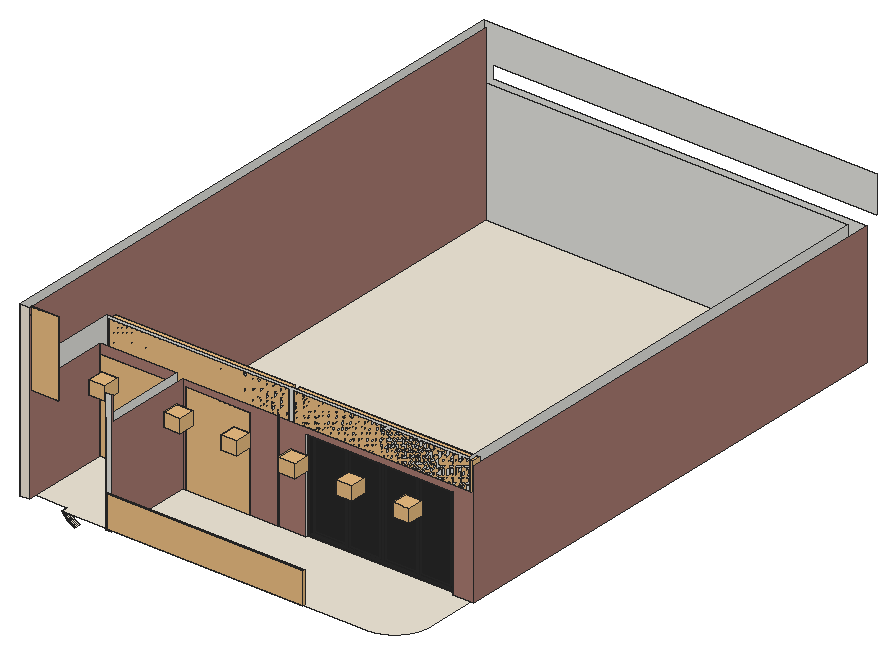
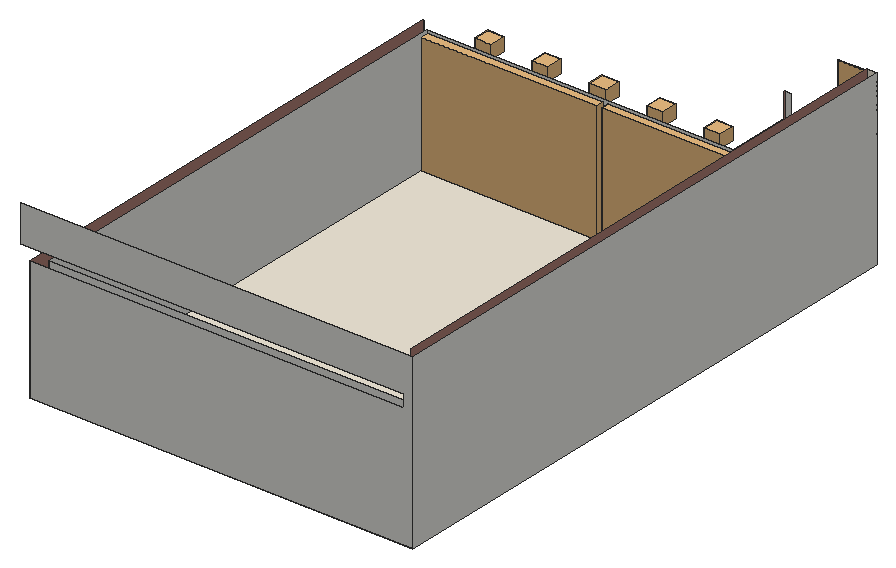
# SketchUp Ruby script. Lengths in inches.
U = 1.inch
M = Sketchup.active_model
def pt(a) = Geom::Point3d.new(a.map { |v| v * U })
def face(e, loops, mat)
  f = e.add_face(loops[0].map { |a| pt(a) })
  loops[1..].each { |l| e.add_face(l.map { |a| pt(a) }).erase! }
  f.material = f.back_material = mat if mat
  f
end
# faces: each face lists its corners as indices into pts; further lists are holes
def faces(e, pts, list, mat = nil) = list.each { |f| face(e, (f[0].is_a?(Array) ? f : [f]).map { |l| l.map { |i| pts[i] } }, mat) }
# xy, xz, yz: faces in a plane at the given z, y or x. An outline is a flat list of corners, or four numbers for a rectangle; further outlines are holes
def ring(l) = l.size == 4 ? [[l[0], l[1]], [l[2], l[1]], [l[2], l[3]], [l[0], l[3]]] : l.each_slice(2).to_a
def flat(e, list, mat, &to3) = list.each { |f| face(e, (f[0].is_a?(Array) ? f : [f]).map { |l| ring(l).map { |u, v| to3.(u, v) } }, mat) }
def xy(e, z, list, mat = nil) = flat(e, list, mat) { |x, y| [x, y, z] }
def xz(e, y, list, mat = nil) = flat(e, list, mat) { |x, z| [x, y, z] }
def yz(e, x, list, mat = nil) = flat(e, list, mat) { |y, z| [x, y, z] }
def lines(e, pts, list) = list.each { |a, b| e.add_line(pt(pts[a]), pt(pts[b])) }
# prism: a flat outline (further loops are holes) pulled along v
def prism(e, loops, v, mat = nil)
  f = face(e, loops, mat); d = Geom::Vector3d.new(v.map { |x| x * U })
  f.pushpull(f.normal.samedirection?(d) ? d.length : -d.length)
end
def box(e, o, s, mat = nil) = prism(e, [[o, [o[0] + s[0], o[1], o[2]], [o[0] + s[0], o[1] + s[1], o[2]], [o[0], o[1] + s[1], o[2]]]], [0, 0, s[2]], mat)
def at(x, y, z, deg = 0) = Geom::Transformation.translation(pt([x, y, z])) * Geom::Transformation.rotation(ORIGIN, Z_AXIS, deg.degrees)
def axes(o, x, y, z) = Geom::Transformation.new([*x, 0, *y, 0, *z, 0, *pt(o).to_a, 1])
def part(name) = M.definitions.add(name)
# library, detail: a bought-in or finely detailed component or shape, given as its bounding box
def library(name, o, s) = part(name).tap { |d| box(d.entities, o, s) }
def detail(e, o, s) = box(e.add_group.entities, o, s)
def put(e, d, t, mat = nil) = e.add_instance(d, t).tap { |i| i.material = mat if mat }
def group(e, t, mat = nil) = e.add_group.tap { |g| g.transformation = t; g.material = mat if mat }.entities
root = M.entities
M.materials.add("0027 AP L140 CRUSHED ICE").color = [241, 233, 217]
M.materials.add("1101 AP 9929 Burnished Earth-N").color = [167, 121, 112]
M.materials.add("False ceiling Light").color = [253, 207, 127]
M.materials.add("[Metal Seamed]").color = [40, 40, 40]
M.materials.add("[Wood Cherry Original]").color = [103, 58, 28]
c1 = library("SLIDING+GLASS+DOOR",[0,-0.75,0],[72,5.75,80])
c2 = library("Curtains",[0,0,0],[121.73,8.19,117.22])
c3 = part("Group\#640")
prism(c3.entities,[[[0,0.08,0],[0,0.08,37.01],[0,0.08,39.37],[0,0.08,76.38],[19.69,0.08,76.38],[19.69,0.08,39.37],[19.69,0.08,37.01],[19.69,0.08,0]]],[0,-0.08,0])
c4 = part("Sliding 4 Door")
g1 = group(c4.entities,at(47.24,2.95,1.58))
put(g1,c3,at(1.57,0.39,1.57))
g2 = group(g1,at(0,0,0))
prism(g2,[[[22.83,0.79,0],[0,0.79,0],[0,0.79,79.53],[22.83,0.79,79.53]],[[21.26,0.79,77.95],[1.57,0.79,77.95],[1.57,0.79,1.57],[21.26,0.79,1.57]]],[0,-0.79,0],"[Metal Seamed]")
g3 = group(c4.entities,at(24.41,2.17,1.58))
put(g3,c3,at(1.57,0.39,1.57))
g4 = group(g3,at(0,0,0))
prism(g4,[[[22.83,0.79,0],[0,0.79,0],[0,0.79,79.53],[22.83,0.79,79.53],[22.83,0.79,39.37]],[[21.26,0.79,77.95],[1.57,0.79,77.95],[1.57,0.79,1.57],[21.26,0.79,1.57]]],[0,-0.79,0],"[Metal Seamed]")
g5 = group(c4.entities,at(-1.57,0,39.37))
prism(g5,[[[96.46,5.12,43.31],[96.46,5.12,-39.37],[1.57,5.12,-39.37],[1.57,5.12,43.31]],[[3.15,5.12,-37.8],[94.88,5.12,-37.8],[94.88,5.12,41.73],[3.15,5.12,41.73]]],[0,-5.12,0],"[Metal Seamed]")
g6 = group(c4.entities,at(1.57,2.95,1.58))
put(g6,c3,at(1.57,0.39,1.57))
g7 = group(g6,at(0,0,0))
prism(g7,[[[22.83,0.79,0],[0,0.79,0],[0,0.79,79.53],[22.83,0.79,79.53]],[[21.26,0.79,77.95],[1.57,0.79,77.95],[1.57,0.79,1.57],[21.26,0.79,1.57]]],[0,-0.79,0],"[Metal Seamed]")
g8 = group(c4.entities,at(70.08,2.17,1.58))
g9 = group(g8,at(1.57,0.39,1.57))
prism(g9,[[[0,0.08,0],[0,0.08,37.01],[0,0.08,39.37],[0,0.08,76.38],[19.69,0.08,76.38],[19.69,0.08,39.37],[19.69,0.08,37.01],[19.69,0.08,0]]],[0,-0.08,0])
g10 = group(g8,at(0,0,0))
prism(g10,[[[22.83,0.79,0],[0,0.79,0],[0,0.79,79.53],[22.83,0.79,79.53],[22.83,0.79,39.37]],[[1.57,0.79,77.95],[1.57,0.79,37.8],[1.57,0.79,1.57],[21.26,0.79,1.57],[21.26,0.79,77.95]]],[0,-0.79,0],"[Metal Seamed]")
c5 = library("Group\#24",[0,0,0],[192,2,30.02])
c6 = library("3",[-5.94,-5.94,-13.08],[15.84,15.84,13.08])
c7 = library("Group\#30",[0,-0.5,0],[27,0.5,73])
xy(root,123,[[59.84,255,59.76,255.01,59.6875,255.02,59.61,255.03,59.45,255.05,59.375,255.07,59.3,255.08,59.22,255.1,59.15,255.125,59.07,255.15,59,255.17,58.92,255.2,58.71,255.29,58.64,255.33,58.57,255.36,58.43,255.44,58.37,255.48,58.3,255.53,58.24,255.57,58.17,255.62,57.93,255.82,57.88,255.88,57.82,255.93,57.62,256.17,57.57,256.24,57.53,256.3,57.48,256.37,57.44,256.43,57.36,256.57,57.33,256.64,57.29,256.71,57.2,256.92,57.17,257,57.15,257.07,57.125,257.15,57.1,257.22,57.08,257.3,57.07,257.375,57.05,257.45,57.03,257.61,57.02,257.6875,57.01,257.76,57,257.84,57,258.16,57.01,258.24,57.02,258.3125,57.03,258.39,57.05,258.55,57.07,258.625,57.08,258.7,57.1,258.78,57.125,258.85,57.15,258.93,57.17,259,57.2,259.08,57.29,259.29,57.33,259.36,57.36,259.43,57.44,259.57,57.48,259.63,57.53,259.7,57.57,259.76,57.62,259.83,57.82,260.07,57.88,260.12,57.93,260.18,58.17,260.38,58.24,260.43,58.3,260.47,58.37,260.52,58.43,260.56,58.57,260.64,58.64,260.67,58.71,260.71,58.92,260.8,59,260.83,59.07,260.85,59.15,260.875,59.22,260.9,59.3,260.92,59.375,260.93,59.45,260.95,59.61,260.97,59.6875,260.98,59.76,260.99,59.84,261,60.16,261,60.24,260.99,60.3125,260.98,60.39,260.97,60.55,260.95,60.625,260.93,60.7,260.92,60.78,260.9,60.85,260.875,60.93,260.85,61,260.83,61.08,260.8,61.29,260.71,61.36,260.67,61.43,260.64,61.57,260.56,61.63,260.52,61.7,260.47,61.76,260.43,61.83,260.38,62.07,260.18,62.12,260.12,62.18,260.07,62.38,259.83,62.43,259.76,62.47,259.7,62.52,259.63,62.56,259.57,62.64,259.43,62.67,259.36,62.71,259.29,62.8,259.08,62.83,259,62.85,258.93,62.875,258.85,62.9,258.78,62.92,258.7,62.93,258.625,62.95,258.55,62.97,258.39,62.98,258.3125,62.99,258.24,63,258.16,63,257.84,62.99,257.76,62.98,257.6875,62.97,257.61,62.95,257.45,62.93,257.375,62.92,257.3,62.9,257.22,62.875,257.15,62.85,257.07,62.83,257,62.8,256.92,62.71,256.71,62.67,256.64,62.64,256.57,62.56,256.43,62.52,256.37,62.47,256.3,62.43,256.24,62.38,256.17,62.18,255.93,62.12,255.88,62.07,255.82,61.83,255.62,61.76,255.57,61.7,255.53,61.63,255.48,61.57,255.44,61.43,255.36,61.36,255.33,61.29,255.29,61.08,255.2,61,255.17,60.93,255.15,60.85,255.125,60.78,255.1,60.7,255.08,60.625,255.07,60.55,255.05,60.39,255.03,60.3125,255.02,60.24,255.01,60.16,255],[122.84,255,122.76,255.01,122.6875,255.02,122.61,255.03,122.45,255.05,122.375,255.07,122.3,255.08,122.22,255.1,122.15,255.125,122.07,255.15,122,255.17,121.92,255.2,121.71,255.29,121.64,255.33,121.57,255.36,121.43,255.44,121.37,255.48,121.3,255.53,121.24,255.57,121.17,255.62,120.93,255.82,120.88,255.88,120.82,255.93,120.62,256.17,120.57,256.24,120.53,256.3,120.48,256.37,120.44,256.43,120.36,256.57,120.33,256.64,120.29,256.71,120.2,256.92,120.17,257,120.15,257.07,120.125,257.15,120.1,257.22,120.08,257.3,120.07,257.375,120.05,257.45,120.03,257.61,120.02,257.6875,120.01,257.76,120,257.84,120,258.16,120.01,258.24,120.02,258.3125,120.03,258.39,120.05,258.55,120.07,258.625,120.08,258.7,120.1,258.78,120.125,258.85,120.15,258.93,120.17,259,120.2,259.08,120.29,259.29,120.33,259.36,120.36,259.43,120.44,259.57,120.48,259.63,120.53,259.7,120.57,259.76,120.62,259.83,120.82,260.07,120.88,260.12,120.93,260.18,121.17,260.38,121.24,260.43,121.3,260.47,121.37,260.52,121.43,260.56,121.57,260.64,121.64,260.67,121.71,260.71,121.92,260.8,122,260.83,122.07,260.85,122.15,260.875,122.22,260.9,122.3,260.92,122.375,260.93,122.45,260.95,122.61,260.97,122.6875,260.98,122.76,260.99,122.84,261,123.16,261,123.24,260.99,123.3125,260.98,123.39,260.97,123.55,260.95,123.625,260.93,123.7,260.92,123.78,260.9,123.85,260.875,123.93,260.85,124,260.83,124.08,260.8,124.29,260.71,124.36,260.67,124.43,260.64,124.57,260.56,124.63,260.52,124.7,260.47,124.76,260.43,124.83,260.38,125.07,260.18,125.12,260.12,125.18,260.07,125.38,259.83,125.43,259.76,125.47,259.7,125.52,259.63,125.56,259.57,125.64,259.43,125.67,259.36,125.71,259.29,125.8,259.08,125.83,259,125.85,258.93,125.875,258.85,125.9,258.78,125.92,258.7,125.93,258.625,125.95,258.55,125.97,258.39,125.98,258.3125,125.99,258.24,126,258.16,126,257.84,125.99,257.76,125.98,257.6875,125.97,257.61,125.95,257.45,125.93,257.375,125.92,257.3,125.9,257.22,125.875,257.15,125.85,257.07,125.83,257,125.8,256.92,125.71,256.71,125.67,256.64,125.64,256.57,125.56,256.43,125.52,256.37,125.47,256.3,125.43,256.24,125.38,256.17,125.18,255.93,125.12,255.88,125.07,255.82,124.83,255.62,124.76,255.57,124.7,255.53,124.63,255.48,124.57,255.44,124.43,255.36,124.36,255.33,124.29,255.29,124.08,255.2,124,255.17,123.93,255.15,123.85,255.125,123.78,255.1,123.7,255.08,123.625,255.07,123.55,255.05,123.39,255.03,123.3125,255.02,123.24,255.01,123.16,255],[185.84,255,185.76,255.01,185.6875,255.02,185.61,255.03,185.45,255.05,185.375,255.07,185.3,255.08,185.22,255.1,185.15,255.125,185.07,255.15,185,255.17,184.92,255.2,184.71,255.29,184.64,255.33,184.57,255.36,184.43,255.44,184.37,255.48,184.3,255.53,184.24,255.57,184.17,255.62,183.93,255.82,183.88,255.88,183.82,255.93,183.62,256.17,183.57,256.24,183.53,256.3,183.48,256.37,183.44,256.43,183.36,256.57,183.33,256.64,183.29,256.71,183.2,256.92,183.17,257,183.15,257.07,183.125,257.15,183.1,257.22,183.08,257.3,183.07,257.375,183.05,257.45,183.03,257.61,183.02,257.6875,183.01,257.76,183,257.84,183,258.16,183.01,258.24,183.02,258.3125,183.03,258.39,183.05,258.55,183.07,258.625,183.08,258.7,183.1,258.78,183.125,258.85,183.15,258.93,183.17,259,183.2,259.08,183.29,259.29,183.33,259.36,183.36,259.43,183.44,259.57,183.48,259.63,183.53,259.7,183.57,259.76,183.62,259.83,183.82,260.07,183.88,260.12,183.93,260.18,184.17,260.38,184.24,260.43,184.3,260.47,184.37,260.52,184.43,260.56,184.57,260.64,184.64,260.67,184.71,260.71,184.92,260.8,185,260.83,185.07,260.85,185.15,260.875,185.22,260.9,185.3,260.92,185.375,260.93,185.45,260.95,185.61,260.97,185.6875,260.98,185.76,260.99,185.84,261,186.16,261,186.24,260.99,186.3125,260.98,186.39,260.97,186.55,260.95,186.625,260.93,186.7,260.92,186.78,260.9,186.85,260.875,186.93,260.85,187,260.83,187.08,260.8,187.29,260.71,187.36,260.67,187.43,260.64,187.57,260.56,187.63,260.52,187.7,260.47,187.76,260.43,187.83,260.38,188.07,260.18,188.12,260.12,188.18,260.07,188.38,259.83,188.43,259.76,188.47,259.7,188.52,259.63,188.56,259.57,188.64,259.43,188.67,259.36,188.71,259.29,188.8,259.08,188.83,259,188.85,258.93,188.875,258.85,188.9,258.78,188.92,258.7,188.93,258.625,188.95,258.55,188.97,258.39,188.98,258.3125,188.99,258.24,189,258.16,189,257.84,188.99,257.76,188.98,257.6875,188.97,257.61,188.95,257.45,188.93,257.375,188.92,257.3,188.9,257.22,188.875,257.15,188.85,257.07,188.83,257,188.8,256.92,188.71,256.71,188.67,256.64,188.64,256.57,188.56,256.43,188.52,256.37,188.47,256.3,188.43,256.24,188.38,256.17,188.18,255.93,188.12,255.88,188.07,255.82,187.83,255.62,187.76,255.57,187.7,255.53,187.63,255.48,187.57,255.44,187.43,255.36,187.36,255.33,187.29,255.29,187.08,255.2,187,255.17,186.93,255.15,186.85,255.125,186.78,255.1,186.7,255.08,186.625,255.07,186.55,255.05,186.39,255.03,186.3125,255.02,186.24,255.01,186.16,255],[248.84,255,248.76,255.01,248.6875,255.02,248.61,255.03,248.45,255.05,248.375,255.07,248.3,255.08,248.22,255.1,248.15,255.125,248.07,255.15,248,255.17,247.92,255.2,247.71,255.29,247.64,255.33,247.57,255.36,247.43,255.44,247.37,255.48,247.3,255.53,247.24,255.57,247.17,255.62,246.93,255.82,246.88,255.88,246.82,255.93,246.62,256.17,246.57,256.24,246.53,256.3,246.48,256.37,246.44,256.43,246.36,256.57,246.33,256.64,246.29,256.71,246.2,256.92,246.17,257,246.15,257.07,246.125,257.15,246.1,257.22,246.08,257.3,246.07,257.375,246.05,257.45,246.03,257.61,246.02,257.6875,246.01,257.76,246,257.84,246,258.16,246.01,258.24,246.02,258.3125,246.03,258.39,246.05,258.55,246.07,258.625,246.08,258.7,246.1,258.78,246.125,258.85,246.15,258.93,246.17,259,246.2,259.08,246.29,259.29,246.33,259.36,246.36,259.43,246.44,259.57,246.48,259.63,246.53,259.7,246.57,259.76,246.62,259.83,246.82,260.07,246.88,260.12,246.93,260.18,247.17,260.38,247.24,260.43,247.3,260.47,247.37,260.52,247.43,260.56,247.57,260.64,247.64,260.67,247.71,260.71,247.92,260.8,248,260.83,248.07,260.85,248.15,260.875,248.22,260.9,248.3,260.92,248.375,260.93,248.45,260.95,248.61,260.97,248.6875,260.98,248.76,260.99,248.84,261,249.16,261,249.24,260.99,249.3125,260.98,249.39,260.97,249.55,260.95,249.625,260.93,249.7,260.92,249.78,260.9,249.85,260.875,249.93,260.85,250,260.83,250.08,260.8,250.29,260.71,250.36,260.67,250.43,260.64,250.57,260.56,250.63,260.52,250.7,260.47,250.76,260.43,250.83,260.38,251.07,260.18,251.12,260.12,251.18,260.07,251.38,259.83,251.43,259.76,251.47,259.7,251.52,259.63,251.56,259.57,251.64,259.43,251.67,259.36,251.71,259.29,251.8,259.08,251.83,259,251.85,258.93,251.875,258.85,251.9,258.78,251.92,258.7,251.93,258.625,251.95,258.55,251.97,258.39,251.98,258.3125,251.99,258.24,252,258.16,252,257.84,251.99,257.76,251.98,257.6875,251.97,257.61,251.95,257.45,251.93,257.375,251.92,257.3,251.9,257.22,251.875,257.15,251.85,257.07,251.83,257,251.8,256.92,251.71,256.71,251.67,256.64,251.64,256.57,251.56,256.43,251.52,256.37,251.47,256.3,251.43,256.24,251.38,256.17,251.18,255.93,251.12,255.88,251.07,255.82,250.83,255.62,250.76,255.57,250.7,255.53,250.63,255.48,250.57,255.44,250.43,255.36,250.36,255.33,250.29,255.29,250.08,255.2,250,255.17,249.93,255.15,249.85,255.125,249.78,255.1,249.7,255.08,249.625,255.07,249.55,255.05,249.39,255.03,249.3125,255.02,249.24,255.01,249.16,255],[311.84,255,311.76,255.01,311.6875,255.02,311.61,255.03,311.45,255.05,311.375,255.07,311.3,255.08,311.22,255.1,311.15,255.125,311.07,255.15,311,255.17,310.92,255.2,310.71,255.29,310.64,255.33,310.57,255.36,310.43,255.44,310.37,255.48,310.3,255.53,310.24,255.57,310.17,255.62,309.93,255.82,309.88,255.88,309.82,255.93,309.62,256.17,309.57,256.24,309.53,256.3,309.48,256.37,309.44,256.43,309.36,256.57,309.33,256.64,309.29,256.71,309.2,256.92,309.17,257,309.15,257.07,309.125,257.15,309.1,257.22,309.08,257.3,309.07,257.375,309.05,257.45,309.03,257.61,309.02,257.6875,309.01,257.76,309,257.84,309,258.16,309.01,258.24,309.02,258.3125,309.03,258.39,309.05,258.55,309.07,258.625,309.08,258.7,309.1,258.78,309.125,258.85,309.15,258.93,309.17,259,309.2,259.08,309.29,259.29,309.33,259.36,309.36,259.43,309.44,259.57,309.48,259.63,309.53,259.7,309.57,259.76,309.62,259.83,309.82,260.07,309.88,260.12,309.93,260.18,310.17,260.38,310.24,260.43,310.3,260.47,310.37,260.52,310.43,260.56,310.57,260.64,310.64,260.67,310.71,260.71,310.92,260.8,311,260.83,311.07,260.85,311.15,260.875,311.22,260.9,311.3,260.92,311.375,260.93,311.45,260.95,311.61,260.97,311.6875,260.98,311.76,260.99,311.84,261,312.16,261,312.24,260.99,312.3125,260.98,312.39,260.97,312.55,260.95,312.625,260.93,312.7,260.92,312.78,260.9,312.85,260.875,312.93,260.85,313,260.83,313.08,260.8,313.29,260.71,313.36,260.67,313.43,260.64,313.57,260.56,313.63,260.52,313.7,260.47,313.76,260.43,313.83,260.38,314.07,260.18,314.12,260.12,314.18,260.07,314.38,259.83,314.43,259.76,314.47,259.7,314.52,259.63,314.56,259.57,314.64,259.43,314.67,259.36,314.71,259.29,314.8,259.08,314.83,259,314.85,258.93,314.875,258.85,314.9,258.78,314.92,258.7,314.93,258.625,314.95,258.55,314.97,258.39,314.98,258.3125,314.99,258.24,315,258.16,315,257.84,314.99,257.76,314.98,257.6875,314.97,257.61,314.95,257.45,314.93,257.375,314.92,257.3,314.9,257.22,314.875,257.15,314.85,257.07,314.83,257,314.8,256.92,314.71,256.71,314.67,256.64,314.64,256.57,314.56,256.43,314.52,256.37,314.47,256.3,314.43,256.24,314.38,256.17,314.18,255.93,314.12,255.88,314.07,255.82,313.83,255.62,313.76,255.57,313.7,255.53,313.63,255.48,313.57,255.44,313.43,255.36,313.36,255.33,313.29,255.29,313.08,255.2,313,255.17,312.93,255.15,312.85,255.125,312.78,255.1,312.7,255.08,312.625,255.07,312.55,255.05,312.39,255.03,312.3125,255.02,312.24,255.01,312.16,255],
  [59.84,333,59.76,333.01,59.6875,333.02,59.61,333.03,59.45,333.05,59.375,333.07,59.3,333.08,59.22,333.1,59.15,333.125,59.07,333.15,59,333.17,58.92,333.2,58.71,333.29,58.64,333.33,58.57,333.36,58.43,333.44,58.37,333.48,58.3,333.53,58.24,333.57,58.17,333.62,57.93,333.82,57.88,333.88,57.82,333.93,57.62,334.17,57.57,334.24,57.53,334.3,57.48,334.37,57.44,334.43,57.36,334.57,57.33,334.64,57.29,334.71,57.2,334.92,57.17,335,57.15,335.07,57.125,335.15,57.1,335.22,57.08,335.3,57.07,335.375,57.05,335.45,57.03,335.61,57.02,335.6875,57.01,335.76,57,335.84,57,336.16,57.01,336.24,57.02,336.3125,57.03,336.39,57.05,336.55,57.07,336.625,57.08,336.7,57.1,336.78,57.125,336.85,57.15,336.93,57.17,337,57.2,337.08,57.29,337.29,57.33,337.36,57.36,337.43,57.44,337.57,57.48,337.63,57.53,337.7,57.57,337.76,57.62,337.83,57.82,338.07,57.88,338.12,57.93,338.18,58.17,338.38,58.24,338.43,58.3,338.47,58.37,338.52,58.43,338.56,58.57,338.64,58.64,338.67,58.71,338.71,58.92,338.8,59,338.83,59.07,338.85,59.15,338.875,59.22,338.9,59.3,338.92,59.375,338.93,59.45,338.95,59.61,338.97,59.6875,338.98,59.76,338.99,59.84,339,60.16,339,60.24,338.99,60.3125,338.98,60.39,338.97,60.55,338.95,60.625,338.93,60.7,338.92,60.78,338.9,60.85,338.875,60.93,338.85,61,338.83,61.08,338.8,61.29,338.71,61.36,338.67,61.43,338.64,61.57,338.56,61.63,338.52,61.7,338.47,61.76,338.43,61.83,338.38,62.07,338.18,62.12,338.12,62.18,338.07,62.38,337.83,62.43,337.76,62.47,337.7,62.52,337.63,62.56,337.57,62.64,337.43,62.67,337.36,62.71,337.29,62.8,337.08,62.83,337,62.85,336.93,62.875,336.85,62.9,336.78,62.92,336.7,62.93,336.625,62.95,336.55,62.97,336.39,62.98,336.3125,62.99,336.24,63,336.16,63,335.84,62.99,335.76,62.98,335.6875,62.97,335.61,62.95,335.45,62.93,335.375,62.92,335.3,62.9,335.22,62.875,335.15,62.85,335.07,62.83,335,62.8,334.92,62.71,334.71,62.67,334.64,62.64,334.57,62.56,334.43,62.52,334.37,62.47,334.3,62.43,334.24,62.38,334.17,62.18,333.93,62.12,333.88,62.07,333.82,61.83,333.62,61.76,333.57,61.7,333.53,61.63,333.48,61.57,333.44,61.43,333.36,61.36,333.33,61.29,333.29,61.08,333.2,61,333.17,60.93,333.15,60.85,333.125,60.78,333.1,60.7,333.08,60.625,333.07,60.55,333.05,60.39,333.03,60.3125,333.02,60.24,333.01,60.16,333],[122.84,333,122.76,333.01,122.6875,333.02,122.61,333.03,122.45,333.05,122.375,333.07,122.3,333.08,122.22,333.1,122.15,333.125,122.07,333.15,122,333.17,121.92,333.2,121.71,333.29,121.64,333.33,121.57,333.36,121.43,333.44,121.37,333.48,121.3,333.53,121.24,333.57,121.17,333.62,120.93,333.82,120.88,333.88,120.82,333.93,120.62,334.17,120.57,334.24,120.53,334.3,120.48,334.37,120.44,334.43,120.36,334.57,120.33,334.64,120.29,334.71,120.2,334.92,120.17,335,120.15,335.07,120.125,335.15,120.1,335.22,120.08,335.3,120.07,335.375,120.05,335.45,120.03,335.61,120.02,335.6875,120.01,335.76,120,335.84,120,336.16,120.01,336.24,120.02,336.3125,120.03,336.39,120.05,336.55,120.07,336.625,120.08,336.7,120.1,336.78,120.125,336.85,120.15,336.93,120.17,337,120.2,337.08,120.29,337.29,120.33,337.36,120.36,337.43,120.44,337.57,120.48,337.63,120.53,337.7,120.57,337.76,120.62,337.83,120.82,338.07,120.88,338.12,120.93,338.18,121.17,338.38,121.24,338.43,121.3,338.47,121.37,338.52,121.43,338.56,121.57,338.64,121.64,338.67,121.71,338.71,121.92,338.8,122,338.83,122.07,338.85,122.15,338.875,122.22,338.9,122.3,338.92,122.375,338.93,122.45,338.95,122.61,338.97,122.6875,338.98,122.76,338.99,122.84,339,123.16,339,123.24,338.99,123.3125,338.98,123.39,338.97,123.55,338.95,123.625,338.93,123.7,338.92,123.78,338.9,123.85,338.875,123.93,338.85,124,338.83,124.08,338.8,124.29,338.71,124.36,338.67,124.43,338.64,124.57,338.56,124.63,338.52,124.7,338.47,124.76,338.43,124.83,338.38,125.07,338.18,125.12,338.12,125.18,338.07,125.38,337.83,125.43,337.76,125.47,337.7,125.52,337.63,125.56,337.57,125.64,337.43,125.67,337.36,125.71,337.29,125.8,337.08,125.83,337,125.85,336.93,125.875,336.85,125.9,336.78,125.92,336.7,125.93,336.625,125.95,336.55,125.97,336.39,125.98,336.3125,125.99,336.24,126,336.16,126,335.84,125.99,335.76,125.98,335.6875,125.97,335.61,125.95,335.45,125.93,335.375,125.92,335.3,125.9,335.22,125.875,335.15,125.85,335.07,125.83,335,125.8,334.92,125.71,334.71,125.67,334.64,125.64,334.57,125.56,334.43,125.52,334.37,125.47,334.3,125.43,334.24,125.38,334.17,125.18,333.93,125.12,333.88,125.07,333.82,124.83,333.62,124.76,333.57,124.7,333.53,124.63,333.48,124.57,333.44,124.43,333.36,124.36,333.33,124.29,333.29,124.08,333.2,124,333.17,123.93,333.15,123.85,333.125,123.78,333.1,123.7,333.08,123.625,333.07,123.55,333.05,123.39,333.03,123.3125,333.02,123.24,333.01,123.16,333],[59.84,411,59.76,411.01,59.6875,411.02,59.61,411.03,59.45,411.05,59.375,411.07,59.3,411.08,59.22,411.1,59.15,411.125,59.07,411.15,59,411.17,58.92,411.2,58.71,411.29,58.64,411.33,58.57,411.36,58.43,411.44,58.37,411.48,58.3,411.53,58.24,411.57,58.17,411.62,57.93,411.82,57.88,411.88,57.82,411.93,57.62,412.17,57.57,412.24,57.53,412.3,57.48,412.37,57.44,412.43,57.36,412.57,57.33,412.64,57.29,412.71,57.2,412.92,57.17,413,57.15,413.07,57.125,413.15,57.1,413.22,57.08,413.3,57.07,413.375,57.05,413.45,57.03,413.61,57.02,413.6875,57.01,413.76,57,413.84,57,414.16,57.01,414.24,57.02,414.3125,57.03,414.39,57.05,414.55,57.07,414.625,57.08,414.7,57.1,414.78,57.125,414.85,57.15,414.93,57.17,415,57.2,415.08,57.29,415.29,57.33,415.36,57.36,415.43,57.44,415.57,57.48,415.63,57.53,415.7,57.57,415.76,57.62,415.83,57.82,416.07,57.88,416.12,57.93,416.18,58.17,416.38,58.24,416.43,58.3,416.47,58.37,416.52,58.43,416.56,58.57,416.64,58.64,416.67,58.71,416.71,58.92,416.8,59,416.83,59.07,416.85,59.15,416.875,59.22,416.9,59.3,416.92,59.375,416.93,59.45,416.95,59.61,416.97,59.6875,416.98,59.76,416.99,59.84,417,60.16,417,60.24,416.99,60.3125,416.98,60.39,416.97,60.55,416.95,60.625,416.93,60.7,416.92,60.78,416.9,60.85,416.875,60.93,416.85,61,416.83,61.08,416.8,61.29,416.71,61.36,416.67,61.43,416.64,61.57,416.56,61.63,416.52,61.7,416.47,61.76,416.43,61.83,416.38,62.07,416.18,62.12,416.12,62.18,416.07,62.38,415.83,62.43,415.76,62.47,415.7,62.52,415.63,62.56,415.57,62.64,415.43,62.67,415.36,62.71,415.29,62.8,415.08,62.83,415,62.85,414.93,62.875,414.85,62.9,414.78,62.92,414.7,62.93,414.625,62.95,414.55,62.97,414.39,62.98,414.3125,62.99,414.24,63,414.16,63,413.84,62.99,413.76,62.98,413.6875,62.97,413.61,62.95,413.45,62.93,413.375,62.92,413.3,62.9,413.22,62.875,413.15,62.85,413.07,62.83,413,62.8,412.92,62.71,412.71,62.67,412.64,62.64,412.57,62.56,412.43,62.52,412.37,62.47,412.3,62.43,412.24,62.38,412.17,62.18,411.93,62.12,411.88,62.07,411.82,61.83,411.62,61.76,411.57,61.7,411.53,61.63,411.48,61.57,411.44,61.43,411.36,61.36,411.33,61.29,411.29,61.08,411.2,61,411.17,60.93,411.15,60.85,411.125,60.78,411.1,60.7,411.08,60.625,411.07,60.55,411.05,60.39,411.03,60.3125,411.02,60.24,411.01,60.16,411],[122.84,411,122.76,411.01,122.6875,411.02,122.61,411.03,122.45,411.05,122.375,411.07,122.3,411.08,122.22,411.1,122.15,411.125,122.07,411.15,122,411.17,121.92,411.2,121.71,411.29,121.64,411.33,121.57,411.36,121.43,411.44,121.37,411.48,121.3,411.53,121.24,411.57,121.17,411.62,120.93,411.82,120.88,411.88,120.82,411.93,120.62,412.17,120.57,412.24,120.53,412.3,120.48,412.37,120.44,412.43,120.36,412.57,120.33,412.64,120.29,412.71,120.2,412.92,120.17,413,120.15,413.07,120.125,413.15,120.1,413.22,120.08,413.3,120.07,413.375,120.05,413.45,120.03,413.61,120.02,413.6875,120.01,413.76,120,413.84,120,414.16,120.01,414.24,120.02,414.3125,120.03,414.39,120.05,414.55,120.07,414.625,120.08,414.7,120.1,414.78,120.125,414.85,120.15,414.93,120.17,415,120.2,415.08,120.29,415.29,120.33,415.36,120.36,415.43,120.44,415.57,120.48,415.63,120.53,415.7,120.57,415.76,120.62,415.83,120.82,416.07,120.88,416.12,120.93,416.18,121.17,416.38,121.24,416.43,121.3,416.47,121.37,416.52,121.43,416.56,121.57,416.64,121.64,416.67,121.71,416.71,121.92,416.8,122,416.83,122.07,416.85,122.15,416.875,122.22,416.9,122.3,416.92,122.375,416.93,122.45,416.95,122.61,416.97,122.6875,416.98,122.76,416.99,122.84,417,123.16,417,123.24,416.99,123.3125,416.98,123.39,416.97,123.55,416.95,123.625,416.93,123.7,416.92,123.78,416.9,123.85,416.875,123.93,416.85,124,416.83,124.08,416.8,124.29,416.71,124.36,416.67,124.43,416.64,124.57,416.56,124.63,416.52,124.7,416.47,124.76,416.43,124.83,416.38,125.07,416.18,125.12,416.12,125.18,416.07,125.38,415.83,125.43,415.76,125.47,415.7,125.52,415.63,125.56,415.57,125.64,415.43,125.67,415.36,125.71,415.29,125.8,415.08,125.83,415,125.85,414.93,125.875,414.85,125.9,414.78,125.92,414.7,125.93,414.625,125.95,414.55,125.97,414.39,125.98,414.3125,125.99,414.24,126,414.16,126,413.84,125.99,413.76,125.98,413.6875,125.97,413.61,125.95,413.45,125.93,413.375,125.92,413.3,125.9,413.22,125.875,413.15,125.85,413.07,125.83,413,125.8,412.92,125.71,412.71,125.67,412.64,125.64,412.57,125.56,412.43,125.52,412.37,125.47,412.3,125.43,412.24,125.38,412.17,125.18,411.93,125.12,411.88,125.07,411.82,124.83,411.62,124.76,411.57,124.7,411.53,124.63,411.48,124.57,411.44,124.43,411.36,124.36,411.33,124.29,411.29,124.08,411.2,124,411.17,123.93,411.15,123.85,411.125,123.78,411.1,123.7,411.08,123.625,411.07,123.55,411.05,123.39,411.03,123.3125,411.02,123.24,411.01,123.16,411]],"0027 AP L140 CRUSHED ICE")
xy(root,132,[[93,213,93,300,81,300,81,309,102,309,102,300,99,300,99,213],[9,214,9,780,384,780,384,300,363,300,363,309,372,309,372,771,18,771,18,214],[165,300,165,309,219,309,219,300,192.5,300,192.5,300.5,191.5,300.5,191.5,300]])
xy(root,132,[[9,214,18,214,18,222,48.22,222,48.22,216,345.375,216,345.75,216.01,346.51,216.03,346.88,216.05,347.26,216.07,347.64,216.1,348.01,216.125,348.39,216.16,348.76,216.2,349.14,216.24,349.51,216.28,349.89,216.33,350.26,216.39,350.63,216.44,351,216.5,351.75,216.64,352.12,216.71,352.48,216.79,353.22,216.95,353.59,217.04,353.95,217.13,354.32,217.23,355.04,217.43,355.41,217.54,355.77,217.65,356.125,217.76,356.48,217.88,356.84,218,357.19,218.13,357.55,218.26,357.9,218.39,358.6,218.67,358.95,218.8125,359.3,218.96,359.64,219.11,359.99,219.27,361.01,219.75,361.34,219.92,361.68,220.1,362.01,220.27,362.34,220.45,362.67,220.64,363,220.82,363.33,221.01,363.65,221.21,363.97,221.4,364.29,221.6,364.61,221.81,364.92,222.01,365.24,222.23,365.55,222.4375,365.85,222.66,366.16,222.875,366.46,223.1,366.77,223.32,367.06,223.55,367.36,223.79,367.66,224.02,368.24,224.5,368.52,224.75,368.81,225,369.37,225.5,369.64,225.76,369.92,226.02,370.1875,226.28,370.46,226.54,370.72,226.8125,370.98,227.08,371.24,227.36,371.5,227.63,372,228.19,372.25,228.48,372.5,228.76,372.98,229.34,373.21,229.64,373.45,229.94,373.68,230.23,373.9,230.54,374.125,230.84,374.34,231.15,374.5625,231.45,374.77,231.76,374.99,232.08,375.19,232.39,375.4,232.71,375.6,233.03,375.79,233.35,375.99,233.67,376.18,234,376.36,234.33,376.55,234.66,376.73,234.99,376.9,235.32,377.08,235.66,377.25,235.99,377.73,237.01,377.89,237.36,378.04,237.7,378.1875,238.05,378.33,238.4,378.61,239.1,378.74,239.45,378.87,239.81,379,240.16,379.12,240.52,379.24,240.875,379.35,241.23,379.46,241.59,379.57,241.96,379.77,242.68,379.87,243.05,379.96,243.41,380.05,243.78,380.21,244.52,380.29,244.88,380.36,245.25,380.5,246,380.56,246.37,380.61,246.74,380.67,247.11,380.72,247.49,380.76,247.86,380.8,248.24,380.84,248.61,380.875,248.99,380.9,249.36,380.93,249.74,380.95,250.12,380.97,250.49,380.99,251.25,381,251.625,381,780,9,780]],"0027 AP L140 CRUSHED ICE")
xy(root,222,[[18,300,81,309],[102,300,165,309],[219,300,363,309]])
xz(root,213,[[93,132,99,252]])
xz(root,214,[[9,132,18,300]],"0027 AP L140 CRUSHED ICE")
xz(root,300,[[81,132,93,132,93,231,18,231,18,222,81,222],[99,132,102,132,102,222,165,222,165,132,191.5,132,191.5,228,99,228],[192.5,132,219,132,219,222,363,222,363,132,384,132,384,252,383,252,383,228,192.5,228]],"1101 AP 9929 Burnished Earth-N")
xz(root,300.5,[[191.5,132,192.5,228]])
xz(root,309,[[81,132,81,222,18,222,18,252,372,252,372,132,363,132,363,222,219,222,219,132,165,132,165,222,102,222,102,132]])
xz(root,771,[[18,132,372,252]])
xz(root,780,[[9,132,9,300,393,300,393,264,18,264,18,252,384,252,384,132]])
yz(root,9,[[214,132,780,300]])
yz(root,18,[[300,222,309,222,309,252,216.5,252,216.5,231,300,231]])
yz(root,18,[[214,132,309,132,309,222,300,222,300,231,216.5,231,216.5,252,309,252,309,132,771,132,771,300,214,300]],"1101 AP 9929 Burnished Earth-N")
yz(root,81,[[300,132,309,222]])
yz(root,93,[[213,132,300,231]])
yz(root,99,[[213,132,300,132,300,228,214,228,214,252,213,252]],"1101 AP 9929 Burnished Earth-N")
yz(root,102,[[300,132,309,222]])
yz(root,165,[[300,132,309,222]])
yz(root,191.5,[[300,132,300.5,228]])
yz(root,192.5,[[300,132,300.5,228]])
yz(root,219,[[300,132,309,222]])
yz(root,363,[[300,132,309,222]])
yz(root,372,[[309,132,771,252]])
yz(root,384,[[300,132,780,252]],"1101 AP 9929 Burnished Earth-N")
p = [[60.63,216,121.51],[60.17,216,121.69],[60.17,222,121.69],[60.63,222,121.51],[59.7,216,121.875],[59.7,222,121.875],
  [59.24,216,122.08],[59.24,222,122.08],[58.78,216,122.28],[58.78,222,122.28],[58.33,216,122.5],[58.33,222,122.5],
  [57.88,216,122.73],[57.88,222,122.73],[57.4375,216,122.97],[57.4375,222,122.97],[57,216,123.22],[57,222,123.22],
  [56.57,216,123.47],[56.57,222,123.47],[56.14,216,123.74],[56.14,222,123.74],[55.72,216,124.01],[55.72,222,124.01],
  [55.3,216,124.29],[55.3,222,124.29],[54.89,216,124.58],[54.89,222,124.58],[54.49,216,124.88],[54.49,222,124.88],
  [54.09,216,125.19],[54.09,222,125.19],[53.7,216,125.51],[53.7,222,125.51],[53.32,216,125.83],[53.32,222,125.83],
  [52.94,216,126.16],[52.94,222,126.16],[52.57,216,126.5],[52.57,222,126.5],[52.21,216,126.85],[52.21,222,126.85],
  [51.85,216,127.21],[51.85,222,127.21],[51.51,216,127.57],[51.51,222,127.57],[51.16,216,127.94],[51.16,222,127.94],
  [50.83,216,128.32],[50.83,222,128.32],[50.51,216,128.7],[50.51,222,128.7],[50.19,216,129.09],[50.19,222,129.09],
  [49.88,216,129.49],[49.88,222,129.49],[49.58,216,129.89],[49.58,222,129.89],[49.29,216,130.3],[49.29,222,130.3],
  [49.01,216,130.72],[49.01,222,130.72],[48.74,216,131.14],[48.74,222,131.14],[48.47,216,131.57],[48.47,222,131.57],
  [48.22,216,132],[48.22,222,132]]
faces(root,p,[[0,1,2,3],[1,4,5,2],[4,6,7,5],[6,8,9,7],[8,10,11,9],[10,12,13,11],[12,14,15,13],[14,16,17,15],
  [16,18,19,17],[18,20,21,19],[20,22,23,21],[22,24,25,23],[24,26,27,25],[26,28,29,27],[28,30,31,29],[30,32,33,31],
  [32,34,35,33],[34,36,37,35],[36,38,39,37],[38,40,41,39],[40,42,43,41],[42,44,45,43],[44,46,47,45],[46,48,49,47],
  [48,50,51,49],[50,52,53,51],[52,54,55,53],[54,56,57,55],[56,58,59,57],[58,60,61,59],[60,62,63,61],[62,64,65,63],
  [64,66,67,65]],"0027 AP L140 CRUSHED ICE")
put(root,c1,axes([18,300.75,132],[0.875,0,0],[0,1,0],[0,0,1.125]))
put(root,c2,axes([200.07,309,132],[1.44235,0,0],[0,1,0],[0,0,1]))
put(root,c2,axes([19.58,309,132],[1.44235,0,0],[0,1,0],[0,0,1]))
g11 = group(root,at(191.5,300.5,132),"False ceiling Light")
box(g11,[0,-0.5,0],[1,0.5,96])
put(root,c1,axes([102,300.75,132],[0.875,0,0],[0,1,0],[0,0,1.125]))
put(root,c4,axes([219,302.5,132],[1.51768,0,0],[0,1,0],[0,0,1.08857]),"[Metal Seamed]")
put(root,c5,at(99,207,137.97),"[Metal Seamed]")
put(root,c6,at(127.02,255.02,229.1))
put(root,c6,at(183.02,255.02,229.1))
put(root,c6,at(239.02,255.02,229.1))
put(root,c6,at(295.02,255.02,229.1))
put(root,c6,at(351.02,255.02,229.1))
put(root,c6,at(53.52,255.02,231.95))
put(root,c7,at(18,216.5,227),"[Wood Cherry Original]")
